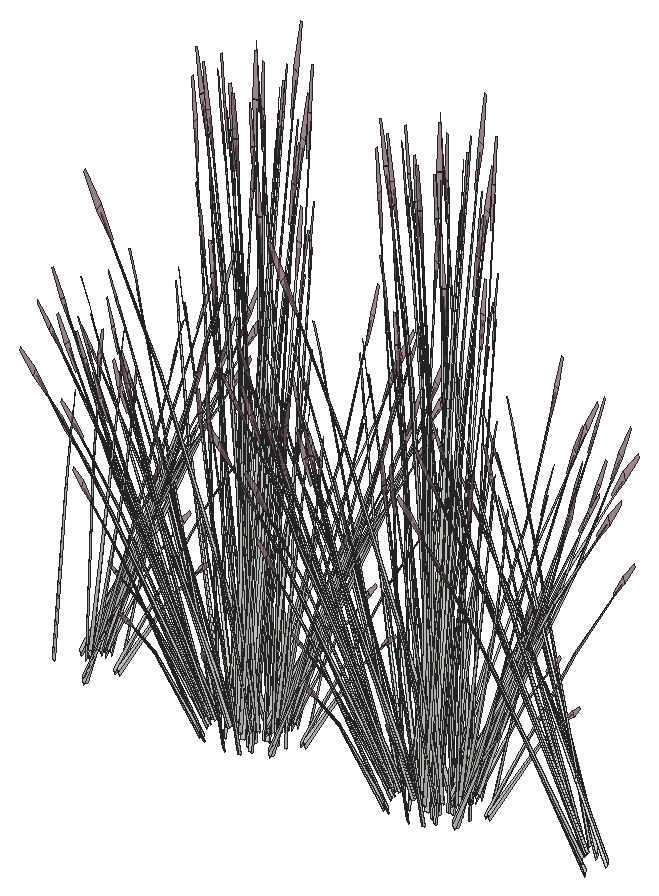
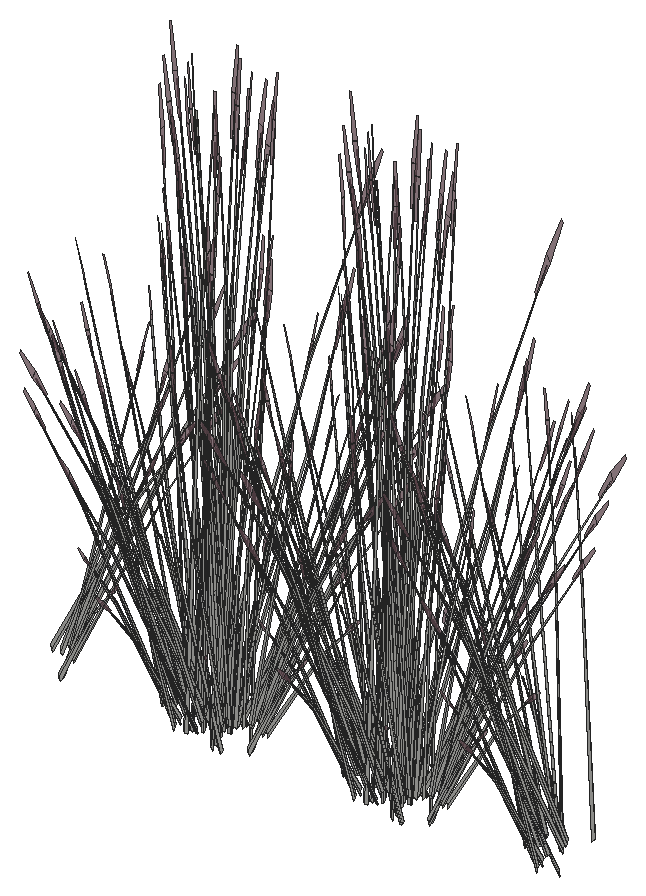
# SketchUp Ruby script. Lengths in inches.
U = 1.inch
M = Sketchup.active_model
def pt(a) = Geom::Point3d.new(a.map { |v| v * U })
def face(e, loops, mat)
  f = e.add_face(loops[0].map { |a| pt(a) })
  loops[1..].each { |l| e.add_face(l.map { |a| pt(a) }).erase! }
  f.material = f.back_material = mat if mat
  f
end
# faces: each face lists its corners as indices into pts; further lists are holes
def faces(e, pts, list, mat = nil) = list.each { |f| face(e, (f[0].is_a?(Array) ? f : [f]).map { |l| l.map { |i| pts[i] } }, mat) }
# xy, xz, yz: faces in a plane at the given z, y or x. An outline is a flat list of corners, or four numbers for a rectangle; further outlines are holes
def ring(l) = l.size == 4 ? [[l[0], l[1]], [l[2], l[1]], [l[2], l[3]], [l[0], l[3]]] : l.each_slice(2).to_a
def flat(e, list, mat, &to3) = list.each { |f| face(e, (f[0].is_a?(Array) ? f : [f]).map { |l| ring(l).map { |u, v| to3.(u, v) } }, mat) }
def xy(e, z, list, mat = nil) = flat(e, list, mat) { |x, y| [x, y, z] }
def xz(e, y, list, mat = nil) = flat(e, list, mat) { |x, z| [x, y, z] }
def yz(e, x, list, mat = nil) = flat(e, list, mat) { |y, z| [x, y, z] }
def lines(e, pts, list) = list.each { |a, b| e.add_line(pt(pts[a]), pt(pts[b])) }
# prism: a flat outline (further loops are holes) pulled along v
def prism(e, loops, v, mat = nil)
  f = face(e, loops, mat); d = Geom::Vector3d.new(v.map { |x| x * U })
  f.pushpull(f.normal.samedirection?(d) ? d.length : -d.length)
end
def box(e, o, s, mat = nil) = prism(e, [[o, [o[0] + s[0], o[1], o[2]], [o[0] + s[0], o[1] + s[1], o[2]], [o[0], o[1] + s[1], o[2]]]], [0, 0, s[2]], mat)
def at(x, y, z, deg = 0) = Geom::Transformation.translation(pt([x, y, z])) * Geom::Transformation.rotation(ORIGIN, Z_AXIS, deg.degrees)
def axes(o, x, y, z) = Geom::Transformation.new([*x, 0, *y, 0, *z, 0, *pt(o).to_a, 1])
def part(name) = M.definitions.add(name)
# library, detail: a bought-in or finely detailed component or shape, given as its bounding box
def library(name, o, s) = part(name).tap { |d| box(d.entities, o, s) }
def detail(e, o, s) = box(e.add_group.entities, o, s)
def put(e, d, t, mat = nil) = e.add_instance(d, t).tap { |i| i.material = mat if mat }
def group(e, t, mat = nil) = e.add_group.tap { |g| g.transformation = t; g.material = mat if mat }.entities
root = M.entities
M.materials.add("LightPink_Translucent").color = [144, 107, 117]
M.materials["LightPink_Translucent"].alpha = 0.75
c1 = part("blade")
p = [[2.15,0.21,22],[0,0.17,0],[0.09,0.45,0],[2.18,0.31,22],[2.29,0.31,22],[0.38,0.45,0],
  [2.48,0.24,33],[2.49,0.24,33],[2.48,0.22,33]]
faces(c1.entities,p,[[0,1,2,3],[4,5,2,3],[6,3,4,7],[8,0,3,6]])
c2 = part("seeds")
p = [[0.3,-0.1,1.38],[-0.01,-0.03,1.59],[-0.01,-0.03,0.03],[0.14,-0.07,-0.07],[0.29,-0.03,3],[0.15,0.01,3.11]]
faces(c2.entities,p,[[0,1,2,3],[1,0,4,5]],"LightPink_Translucent")
c3 = part("blade with seeds")
put(c3.entities,c1,at(0,0,0))
put(c3.entities,c2,axes([2.4,0.25,30.99],[1.5799,-0.05474,1.17369],[-0.12525,1.92788,0.29478],[-0.07173,-0.02425,1.56792]))
put(root,c3,axes([312.2,55.57,257.77],[-0.4278,-0.1757,1.1486],[0.5524,-0.17852,0.84392],[0.14899,0.15122,0.25299]))
put(root,c3,axes([310.68,55.38,257.59],[0.01341,-0.20255,1.43002],[0.64074,-0.22625,-0.30754],[0.1978,0.24243,0.61141]))
put(root,c3,axes([312.27,56.37,257.67],[-0.48723,-0.01916,1.0506],[0.32177,-0.40701,0.58006],[0.19248,0.1446,0.8241]))
put(root,c3,axes([310.8,51.49,258.875],[-0.14147,0.21002,1.71376],[-0.59349,-0.43464,0.13857],[0.26773,-0.27089,0.73262]))
put(root,c3,axes([311.24,55.8125,259.68],[0.74975,-0.14525,-0.51099],[0.13115,0.55007,-0.3958],[0.20138,0.15763,0.97773]))
put(root,c3,axes([312.7,52.53,259.68],[-0.19519,-0.55794,-0.51099],[0.73919,-0.0976,-0.3958],[0.21183,-0.14986,0.97773]))
put(root,c3,axes([314,55.41,258.93],[-0.14542,-0.51365,-0.03492],[0.68734,-0.11809,-0.15832],[0.14353,0.03256,0.52218]))
put(root,c3,axes([324.4375,52.72,258.875],[0.31515,-0.01384,1.71376],[-0.20907,0.5998,0.13857],[-0.44912,-0.0371,0.73262]))
put(root,c3,axes([313.6,51.42,257.77],[-0.25308,0.31105,1.1486],[-0.21753,-0.4179,0.84392],[0.20902,-0.10472,0.25299]))
put(root,c3,axes([311.16,54.37,258.875],[-0.28223,-0.10528,1.71376],[0.58406,-0.44165,0.13857],[0.36402,0.19924,0.73262]))
put(root,c3,axes([324.57,53.77,258.875],[0.26363,-0.12925,1.71376],[0.22195,0.59723,0.13857],[-0.41388,0.13498,0.73262]))
put(root,c3,axes([313.24,52.59,259.53],[0.66138,-0.08733,-0.35414],[0.17464,0.49921,0.4572],[0.18953,-0.13408,0.87481]))
put(root,c3,axes([323.75,54.79,257.59],[0.26405,0.05016,1.43002],[0.17019,0.51235,-0.30754],[-0.35868,0.0959,0.61141]))
put(root,c3,axes([312.72,52.76,259.98],[0.39688,-0.48213,-0.71045],[0.69548,0.34264,0.08574],[0.23697,-0.17468,1.00501]))
put(root,c3,axes([312.71,55.35,259.53],[0.43232,0.38257,-0.35414],[-0.49364,0.36215,0.4572],[0.25081,0.0551,0.87481]))
put(root,c3,axes([326.08,53.15,258.34],[0.21597,-0.08839,1.77064],[0.07448,0.61717,0.13857],[-0.4678,0.08189,0.63284]))
put(root,c3,axes([325.38,52.16,259.98],[-0.75952,-0.01471,-0.71045],[0.05101,-0.61953,0.08574],[-0.32177,-0.06538,1.00501]))
put(root,c3,axes([324.77,52.31,257.59],[0.14835,0.17012,1.43002],[-0.34183,0.46242,-0.30754],[-0.351,-0.11053,0.61141]))
put(root,c3,axes([313.04,53.77,259.68],[0.20584,-0.55581,-0.51099],[0.70573,0.19051,-0.3958],[0.28414,-0.05097,0.97773]))
put(root,c3,axes([324.16,53.23,259.53],[-0.63144,-0.17046,-0.35414],[0.18417,-0.49731,0.4572],[-0.25423,0.0456,0.87481]))
put(root,c3,axes([314.8125,54.125,257.77],[-0.46945,0.10088,1.1486],[0.22097,-0.4169,0.84392],[0.24904,0.02853,0.25299]))
put(root,c3,axes([325.03,51.75,258.875],[0.28223,0.10528,1.71376],[-0.58406,0.44165,0.13857],[-0.36402,-0.19924,0.73262]))
put(root,c3,axes([313.29,52.3125,257.59],[-0.27143,-0.0181,1.43002],[-0.27808,-0.48551,-0.30754],[0.33346,-0.13735,0.61141]))
put(root,c3,axes([313.47,54.02,259.53],[0.63144,0.17046,-0.35414],[-0.18417,0.49731,0.4572],[0.25423,-0.0456,0.87481]))
put(root,c3,axes([324.59,53.49,259.68],[-0.20584,0.55581,-0.51099],[-0.70573,-0.19051,-0.3958],[-0.28414,0.05097,0.97773]))
put(root,c3,axes([325.125,52.28,259.68],[-0.55171,0.40476,-0.51099],[-0.48318,-0.42758,-0.3958],[-0.28031,-0.06159,0.97773]))
put(root,c3,axes([312.25,55.1,259.98],[0.75952,0.01471,-0.71045],[-0.05101,0.61953,0.08574],[0.32177,0.06538,1.00501]))
put(root,c3,axes([311.75,53.41,258.875],[-0.31515,0.01384,1.71376],[0.20907,-0.5998,0.13857],[0.44912,0.0371,0.73262]))
put(root,c3,axes([323.2,55.86,257.77],[0.31665,-0.27694,1.1486],[0.12495,0.43841,0.84392],[-0.22883,0.0785,0.25299]))
put(root,c3,axes([312.91,53.97,259.98],[0.66765,-0.26986,-0.71045],[0.37208,0.55551,0.08574],[0.32259,-0.0631,1.00501]))
put(root,c3,axes([324.92,51.9,259.53],[-0.43232,-0.38257,-0.35414],[0.49364,-0.36215,0.4572],[-0.25081,-0.0551,0.87481]))
put(root,c3,axes([325.53,54.17,258.875],[0.18977,-0.18775,1.71376],[0.47917,0.50677,0.13857],[-0.32866,0.23079,0.73262]))
put(root,c3,axes([324.39,54.67,259.53],[-0.66138,0.08733,-0.35414],[-0.17464,-0.49921,0.4572],[-0.18953,0.13408,0.87481]))
put(root,c3,axes([323.88,52.82,257.77],[0.48508,-0.04372,1.1486],[-0.3077,0.38525,0.84392],[-0.23971,-0.05779,0.25299]))
put(root,c3,axes([313.93,54.79,257.59],[-0.18299,-0.15028,1.43002],[0.23809,-0.49714,-0.30754],[0.37023,0.06735,0.61141]))
put(root,c3,axes([325.39,54.64,258.875],[0.14147,-0.21002,1.71376],[0.59349,0.43464,0.13857],[-0.26773,0.27089,0.73262]))
put(root,c3,axes([324.94,54.72,259.68],[0.19519,0.55794,-0.51099],[-0.73919,0.0976,-0.3958],[-0.21183,0.14986,0.97773]))
put(root,c3,axes([326.7,51.43,259.98],[-0.64788,-0.29534,-0.71045],[0.46044,-0.51755,0.08574],[-0.23473,-0.17635,1.00501]))
put(root,c3,axes([326.4,51.44,259.68],[-0.74975,0.14525,-0.51099],[-0.13115,-0.55007,-0.3958],[-0.20138,-0.15763,0.97773]))
put(root,c3,axes([325.97,50.625,257.59],[-0.04601,0.19989,1.43002],[-0.67263,0.16733,-0.30754],[-0.15723,-0.25836,0.61141]))
put(root,c3,axes([326.19,51.14,258.875],[0.17368,0.19618,1.71376],[-0.80256,0.16516,0.13857],[-0.18139,-0.30799,0.73262]))
put(root,c3,axes([326.48,51.04,259.53],[-0.11735,-0.49217,-0.35414],[0.67083,-0.12996,0.4572],[-0.18018,-0.14104,0.87481]))
put(root,c3,axes([325.55,55.82,259.53],[-0.5141,0.32171,-0.35414],[-0.48666,-0.36734,0.4572],[-0.07405,0.18664,0.87481]))
put(root,c3,axes([328.25,54.77,258.33],[0.65659,0.2464,1.51261],[-0.64324,0.53082,0.59816],[-0.28812,-0.31461,1.26806]))
put(root,c3,axes([325.74,50.3,257.77],[0.39634,0.21267,1.1486],[-0.57721,0.12784,0.84392],[-0.1235,-0.16344,0.25299]))
put(root,c3,axes([325.88,57.07,257.77],[-0.01966,-0.36332,1.1486],[0.49135,0.25914,0.84392],[-0.09663,0.17317,0.25299]))
put(root,c3,axes([326.58,55.54,257.48],[0.7111,0.30552,0.49651],[-0.42504,0.54784,0],[-0.16196,-0.06958,1.57504]))
put(root,c3,axes([327.6,54.59,257.62],[-0.14658,0.54532,0.1448],[-0.71613,-0.09466,-0.41347],[-0.13033,-0.05599,1.26744]))
put(root,c3,axes([325.18,53.63,257.48],[0,0.61104,0.49651],[-0.85008,0,0],[0,-0.13917,1.57504]))
put(root,c3,axes([326.07,55.67,260],[0.54391,0.41056,-0.5672],[-0.57458,0.35956,-0.43934],[-0.08276,0.2086,1.08528]))
put(root,c3,axes([329.27,53.59,257.84],[-0.02076,-0.57531,1.41272],[0.93937,0.14913,0.59816],[-0.22217,0.31481,1.3335]))
put(root,c3,axes([325.47,56.29,257.82],[0.69024,-0.1082,0.06507],[0.15868,0.43593,-0.86304],[-0.04376,0.22067,0.7736]))
put(root,c3,axes([328.0625,51.1875,259.68],[-0.7469,-0.15318,-0.51099],[0.25601,-0.52518,-0.3958],[-0.06849,-0.21144,0.97773]))
put(root,c3,axes([327.37,54.07,257.36],[0.96033,0.12874,0.45755],[-0.19544,0.7271,0.17955],[-0.14034,-0.07021,1.58856]))
put(root,c3,axes([327.12,53.94,257.72],[-0.36864,0.55059,0.44739],[-0.76598,-0.26498,-0.21531],[0,-0.12692,1.43643]))
put(root,c3,axes([328.33,51.29,259.98],[-0.36264,-0.49684,-0.71045],[0.74649,-0.27689,0.08574],[-0.0848,-0.24006,1.00501]))
put(root,c3,axes([326.85,55.23,257.47],[0.81646,-0.16218,0.17642],[0.20161,0.60355,0.35086],[-0.07282,-0.08794,1.60407]))
put(root,c3,axes([329.28,55.27,257.47],[0.21949,-0.60727,0.17642],[0.8032,0.17185,0.35086],[-0.13875,0.00296,1.60407]))
put(root,c3,axes([328.91,54.46,257.62],[0.56134,0.36712,0.1448],[-0.46823,0.41419,-0.41347],[-0.13033,0.05599,1.26744]))
put(root,c3,axes([328.89,54.19,257.72],[0.82508,-0.03772,0.44739],[0.07462,0.62614,-0.21531],[-0.14771,0.06346,1.43643]))
put(root,c3,axes([329.51,55.59,257.48],[0.7111,-0.30552,0.49651],[0.42504,0.54784,0],[-0.16196,0.06958,1.57504]))
put(root,c3,axes([328.4,50.87,259.53],[0.22906,-0.4699,-0.35414],[0.66828,0.13705,0.4572],[-0.06128,-0.18919,0.87481]))
put(root,c3,axes([327.28,53.4,257.36],[0.33034,0.68327,0.45755],[-0.94388,0.2376,0.17955],[0.01154,-0.12555,1.58856]))
put(root,c3,axes([330.53,53.72,257.47],[-0.59697,-0.44509,0.17642],[0.60159,-0.4317,0.35086],[-0.06593,0.0909,1.60407]))
put(root,c3,axes([327.59,53.59,257.43],[0.8561,0.29616,0.24065],[-0.41201,0.61537,0.50002],[0,-0.14185,1.60543]))
put(root,c3,axes([327.3125,53.18,257.72],[-0.82508,0.03772,0.44739],[-0.07462,-0.62614,-0.21531],[0.14771,-0.06346,1.43643]))
put(root,c3,axes([326.93,52.1,257.47],[-0.21949,0.60727,0.17642],[-0.8032,-0.17185,0.35086],[0.13875,-0.00296,1.60407]))
put(root,c3,axes([329.36,52.14,257.47],[-0.81646,0.16218,0.17642],[-0.20161,-0.60355,0.35086],[0.07282,0.08794,1.60407]))
put(root,c3,axes([328.52,49.875,257.77],[0.09747,0.35631,1.1486],[-0.54071,-0.19735,0.84392],[0.05818,-0.18244,0.25299]))
put(root,c3,axes([328.02,53.02,257.36],[-0.62999,0.55453,0.45755],[-0.74845,-0.4895,0.17955],[0.15188,-0.05534,1.58856]))
put(root,c3,axes([329.09,53.43,257.72],[0.36864,-0.55059,0.44739],[0.76598,0.26498,-0.21531],[0,0.12692,1.43643]))
put(root,c3,axes([327.68,56.07,259.68],[0.7469,0.15318,-0.51099],[-0.25601,0.52518,-0.3958],[0.06849,0.21144,0.97773]))
put(root,c3,axes([328.84,53.3,257.38],[-0.96033,-0.12874,0.49198],[0.19544,-0.7271,0.19306],[0.14034,0.07021,1.70813]))
put(root,c3,axes([328.3,52.92,257.72],[-0.45644,-0.51287,0.44739],[0.69137,-0.36116,-0.21531],[0.14771,0.06346,1.43643]))
put(root,c3,axes([329.41,53.55,257.62],[0.70791,-0.1782,0.1448],[0.24791,0.50885,-0.41347],[0,0.11199,1.26744]))
put(root,c3,axes([329.67,51.59,259.68],[-0.54391,-0.41056,-0.51099],[0.57458,-0.35956,-0.3958],[0.08276,-0.2086,0.97773]))
put(root,c3,axes([329.32,50.86,257.59],[-0.21597,0.12368,1.43002],[-0.64681,-0.21647,-0.30754],[0.1199,-0.26922,0.61141]))
put(root,c3,axes([331.02,53.74,257.48],[0,-0.61104,0.49651],[0.85008,0,0],[0,0.13917,1.57504]))
put(root,c3,axes([328.1,54.98,258.875],[-0.17368,-0.19618,1.71376],[0.80256,-0.16516,0.13857],[0.18139,0.30799,0.73262]))
put(root,c3,axes([328.6,52.78,257.62],[0.14658,-0.54532,0.1448],[0.71613,0.09466,-0.41347],[0.13033,0.05599,1.26744]))
put(root,c3,axes([329.62,51.83,257.48],[-0.7111,-0.30552,0.49651],[0.42504,-0.54784,0],[0.16196,0.06958,1.57504]))
put(root,c3,axes([329.84,51.77,259.98],[0.01977,-0.56521,-0.71045],[0.83252,0.03796,0.08574],[0.08786,-0.23945,1.00501]))
put(root,c3,axes([330.1875,51.43,259.53],[0.5141,-0.32171,-0.35414],[0.48666,0.36734,0.4572],[0.07405,-0.18664,0.87481]))
put(root,c3,axes([330.31,55.57,257.77],[-0.4278,-0.1757,1.1486],[0.5524,-0.17852,0.84392],[0.14899,0.15122,0.25299]))
put(root,c3,axes([328.79,55.38,257.59],[0.01341,-0.20255,1.43002],[0.64074,-0.22625,-0.30754],[0.1978,0.24243,0.61141]))
put(root,c3,axes([330.38,56.37,257.67],[-0.48723,-0.01916,1.0506],[0.32177,-0.40701,0.58006],[0.19248,0.1446,0.8241]))
put(root,c3,axes([328.91,51.49,258.875],[-0.14147,0.21002,1.71376],[-0.59349,-0.43464,0.13857],[0.26773,-0.27089,0.73262]))
put(root,c3,axes([329.34,55.8125,259.68],[0.74975,-0.14525,-0.51099],[0.13115,0.55007,-0.3958],[0.20138,0.15763,0.97773]))
put(root,c3,axes([330.8,52.53,259.68],[-0.19519,-0.55794,-0.51099],[0.73919,-0.0976,-0.3958],[0.21183,-0.14986,0.97773]))
put(root,c3,axes([342.34,52.72,258.875],[0.31515,-0.01384,1.71376],[-0.20907,0.5998,0.13857],[-0.44912,-0.0371,0.73262]))
put(root,c3,axes([332.1,55.41,258.93],[-0.14542,-0.51365,-0.03492],[0.68734,-0.11809,-0.15832],[0.14353,0.03256,0.52218]))
put(root,c3,axes([331.71,51.42,257.77],[-0.25308,0.31105,1.1486],[-0.21753,-0.4179,0.84392],[0.20902,-0.10472,0.25299]))
put(root,c3,axes([342.47,53.77,258.875],[0.26363,-0.12925,1.71376],[0.22195,0.59723,0.13857],[-0.41388,0.13498,0.73262]))
put(root,c3,axes([329.26,54.37,258.875],[-0.28223,-0.10528,1.71376],[0.58406,-0.44165,0.13857],[0.36402,0.19924,0.73262]))
put(root,c3,axes([341.65,54.79,257.59],[0.26405,0.05016,1.43002],[0.17019,0.51235,-0.30754],[-0.35868,0.0959,0.61141]))
put(root,c3,axes([331.35,52.59,259.53],[0.66138,-0.08733,-0.35414],[0.17464,0.49921,0.4572],[0.18953,-0.13408,0.87481]))
put(root,c3,axes([330.82,52.76,259.98],[0.39688,-0.48213,-0.71045],[0.69548,0.34264,0.08574],[0.23697,-0.17468,1.00501]))
put(root,c3,axes([343.99,53.15,258.34],[0.21597,-0.08839,1.77064],[0.07448,0.61717,0.13857],[-0.4678,0.08189,0.63284]))
put(root,c3,axes([330.82,55.35,259.53],[0.43232,0.38257,-0.35414],[-0.49364,0.36215,0.4572],[0.25081,0.0551,0.87481]))
put(root,c3,axes([343.29,52.16,259.98],[-0.75952,-0.01471,-0.71045],[0.05101,-0.61953,0.08574],[-0.32177,-0.06538,1.00501]))
put(root,c3,axes([342.67,52.31,257.59],[0.14835,0.17012,1.43002],[-0.34183,0.46242,-0.30754],[-0.351,-0.11053,0.61141]))
put(root,c3,axes([342.06,53.23,259.53],[-0.63144,-0.17046,-0.35414],[0.18417,-0.49731,0.4572],[-0.25423,0.0456,0.87481]))
put(root,c3,axes([342.9375,51.75,258.875],[0.28223,0.10528,1.71376],[-0.58406,0.44165,0.13857],[-0.36402,-0.19924,0.73262]))
put(root,c3,axes([331.15,53.77,259.68],[0.20584,-0.55581,-0.51099],[0.70573,0.19051,-0.3958],[0.28414,-0.05097,0.97773]))
put(root,c3,axes([332.92,54.125,257.77],[-0.46945,0.10088,1.1486],[0.22097,-0.4169,0.84392],[0.24904,0.02853,0.25299]))
put(root,c3,axes([342.5,53.49,259.68],[-0.20584,0.55581,-0.51099],[-0.70573,-0.19051,-0.3958],[-0.28414,0.05097,0.97773]))
put(root,c3,axes([331.4,52.3125,257.59],[-0.27143,-0.0181,1.43002],[-0.27808,-0.48551,-0.30754],[0.33346,-0.13735,0.61141]))
put(root,c3,axes([331.58,54.02,259.53],[0.63144,0.17046,-0.35414],[-0.18417,0.49731,0.4572],[0.25423,-0.0456,0.87481]))
put(root,c3,axes([343.03,52.28,259.68],[-0.55171,0.40476,-0.51099],[-0.48318,-0.42758,-0.3958],[-0.28031,-0.06159,0.97773]))
put(root,c3,axes([330.36,55.1,259.98],[0.75952,0.01471,-0.71045],[-0.05101,0.61953,0.08574],[0.32177,0.06538,1.00501]))
put(root,c3,axes([341.1,55.86,257.77],[0.31665,-0.27694,1.1486],[0.12495,0.43841,0.84392],[-0.22883,0.0785,0.25299]))
put(root,c3,axes([329.86,53.41,258.875],[-0.31515,0.01384,1.71376],[0.20907,-0.5998,0.13857],[0.44912,0.0371,0.73262]))
put(root,c3,axes([342.83,51.9,259.53],[-0.43232,-0.38257,-0.35414],[0.49364,-0.36215,0.4572],[-0.25081,-0.0551,0.87481]))
put(root,c3,axes([343.4375,54.17,258.875],[0.18977,-0.18775,1.71376],[0.47917,0.50677,0.13857],[-0.32866,0.23079,0.73262]))
put(root,c3,axes([342.3,54.67,259.53],[-0.66138,0.08733,-0.35414],[-0.17464,-0.49921,0.4572],[-0.18953,0.13408,0.87481]))
put(root,c3,axes([331.01,53.97,259.98],[0.66765,-0.26986,-0.71045],[0.37208,0.55551,0.08574],[0.32259,-0.0631,1.00501]))
put(root,c3,axes([341.79,52.82,257.77],[0.48508,-0.04372,1.1486],[-0.3077,0.38525,0.84392],[-0.23971,-0.05779,0.25299]))
put(root,c3,axes([332.04,54.79,257.59],[-0.18299,-0.15028,1.43002],[0.23809,-0.49714,-0.30754],[0.37023,0.06735,0.61141]))
put(root,c3,axes([343.3,54.64,258.875],[0.14147,-0.21002,1.71376],[0.59349,0.43464,0.13857],[-0.26773,0.27089,0.73262]))
put(root,c3,axes([342.84,54.72,259.68],[0.19519,0.55794,-0.51099],[-0.73919,0.0976,-0.3958],[-0.21183,0.14986,0.97773]))
put(root,c3,axes([344.61,51.43,259.98],[-0.64788,-0.29534,-0.71045],[0.46044,-0.51755,0.08574],[-0.23473,-0.17635,1.00501]))
put(root,c3,axes([344.3,51.44,259.68],[-0.74975,0.14525,-0.51099],[-0.13115,-0.55007,-0.3958],[-0.20138,-0.15763,0.97773]))
put(root,c3,axes([343.88,50.625,257.59],[-0.04601,0.19989,1.43002],[-0.67263,0.16733,-0.30754],[-0.15723,-0.25836,0.61141]))
put(root,c3,axes([344.1,51.14,258.875],[0.17368,0.19618,1.71376],[-0.80256,0.16516,0.13857],[-0.18139,-0.30799,0.73262]))
put(root,c3,axes([344.38,51.04,259.53],[-0.11735,-0.49217,-0.35414],[0.67083,-0.12996,0.4572],[-0.18018,-0.14104,0.87481]))
put(root,c3,axes([343.46,55.82,259.53],[-0.5141,0.32171,-0.35414],[-0.48666,-0.36734,0.4572],[-0.07405,0.18664,0.87481]))
put(root,c3,axes([346.16,54.77,258.33],[0.65659,0.2464,1.51261],[-0.64324,0.53082,0.59816],[-0.28812,-0.31461,1.26806]))
put(root,c3,axes([343.65,50.3,257.77],[0.39634,0.21267,1.1486],[-0.57721,0.12784,0.84392],[-0.1235,-0.16344,0.25299]))
put(root,c3,axes([343.79,57.07,257.77],[-0.01966,-0.36332,1.1486],[0.49135,0.25914,0.84392],[-0.09663,0.17317,0.25299]))
put(root,c3,axes([344.49,55.54,257.48],[0.7111,0.30552,0.49651],[-0.42504,0.54784,0],[-0.16196,-0.06958,1.57504]))
put(root,c3,axes([345.51,54.59,257.62],[-0.14658,0.54532,0.1448],[-0.71613,-0.09466,-0.41347],[-0.13033,-0.05599,1.26744]))
put(root,c3,axes([343.09,53.63,257.48],[0,0.61104,0.49651],[-0.85008,0,0],[0,-0.13917,1.57504]))
put(root,c3,axes([343.97,55.67,260],[0.54391,0.41056,-0.5672],[-0.57458,0.35956,-0.43934],[-0.08276,0.2086,1.08528]))
put(root,c3,axes([347.17,53.59,257.84],[-0.02076,-0.57531,1.41272],[0.93937,0.14913,0.59816],[-0.22217,0.31481,1.3335]))
put(root,c3,axes([343.38,56.29,257.82],[0.69024,-0.1082,0.06507],[0.15868,0.43593,-0.86304],[-0.04376,0.22067,0.7736]))
put(root,c3,axes([345.97,51.1875,259.68],[-0.7469,-0.15318,-0.51099],[0.25601,-0.52518,-0.3958],[-0.06849,-0.21144,0.97773]))
put(root,c3,axes([345.27,54.07,257.36],[0.96033,0.12874,0.45755],[-0.19544,0.7271,0.17955],[-0.14034,-0.07021,1.58856]))
put(root,c3,axes([345.02,53.94,257.72],[-0.36864,0.55059,0.44739],[-0.76598,-0.26498,-0.21531],[0,-0.12692,1.43643]))
put(root,c3,axes([346.24,51.29,259.98],[-0.36264,-0.49684,-0.71045],[0.74649,-0.27689,0.08574],[-0.0848,-0.24006,1.00501]))
put(root,c3,axes([344.76,55.23,257.47],[0.81646,-0.16218,0.17642],[0.20161,0.60355,0.35086],[-0.07282,-0.08794,1.60407]))
put(root,c3,axes([347.1875,55.27,257.47],[0.21949,-0.60727,0.17642],[0.8032,0.17185,0.35086],[-0.13875,0.00296,1.60407]))
put(root,c3,axes([346.81,54.46,257.62],[0.56134,0.36712,0.1448],[-0.46823,0.41419,-0.41347],[-0.13033,0.05599,1.26744]))
put(root,c3,axes([346.8,54.19,257.72],[0.82508,-0.03772,0.44739],[0.07462,0.62614,-0.21531],[-0.14771,0.06346,1.43643]))
put(root,c3,axes([347.41,55.59,257.48],[0.7111,-0.30552,0.49651],[0.42504,0.54784,0],[-0.16196,0.06958,1.57504]))
put(root,c3,axes([346.31,50.87,259.53],[0.22906,-0.4699,-0.35414],[0.66828,0.13705,0.4572],[-0.06128,-0.18919,0.87481]))
put(root,c3,axes([345.1875,53.4,257.36],[0.33034,0.68327,0.45755],[-0.94388,0.2376,0.17955],[0.01154,-0.12555,1.58856]))
put(root,c3,axes([348.4375,53.72,257.47],[-0.59697,-0.44509,0.17642],[0.60159,-0.4317,0.35086],[-0.06593,0.0909,1.60407]))
put(root,c3,axes([345.49,53.59,257.43],[0.8561,0.29616,0.24065],[-0.41201,0.61537,0.50002],[0,-0.14185,1.60543]))
put(root,c3,axes([345.22,53.18,257.72],[-0.82508,0.03772,0.44739],[-0.07462,-0.62614,-0.21531],[0.14771,-0.06346,1.43643]))
put(root,c3,axes([344.83,52.1,257.47],[-0.21949,0.60727,0.17642],[-0.8032,-0.17185,0.35086],[0.13875,-0.00296,1.60407]))
put(root,c3,axes([347.26,52.14,257.47],[-0.81646,0.16218,0.17642],[-0.20161,-0.60355,0.35086],[0.07282,0.08794,1.60407]))
put(root,c3,axes([346.43,49.875,257.77],[0.09747,0.35631,1.1486],[-0.54071,-0.19735,0.84392],[0.05818,-0.18244,0.25299]))
put(root,c3,axes([345.93,53.02,257.36],[-0.62999,0.55453,0.45755],[-0.74845,-0.4895,0.17955],[0.15188,-0.05534,1.58856]))
put(root,c3,axes([347,53.43,257.72],[0.36864,-0.55059,0.44739],[0.76598,0.26498,-0.21531],[0,0.12692,1.43643]))
put(root,c3,axes([345.58,56.07,259.68],[0.7469,0.15318,-0.51099],[-0.25601,0.52518,-0.3958],[0.06849,0.21144,0.97773]))
put(root,c3,axes([346.75,53.3,257.38],[-0.96033,-0.12874,0.49198],[0.19544,-0.7271,0.19306],[0.14034,0.07021,1.70813]))
put(root,c3,axes([346.2,52.92,257.72],[-0.45644,-0.51287,0.44739],[0.69137,-0.36116,-0.21531],[0.14771,0.06346,1.43643]))
put(root,c3,axes([347.32,53.55,257.62],[0.70791,-0.1782,0.1448],[0.24791,0.50885,-0.41347],[0,0.11199,1.26744]))
put(root,c3,axes([347.58,51.59,259.68],[-0.54391,-0.41056,-0.51099],[0.57458,-0.35956,-0.3958],[0.08276,-0.2086,0.97773]))
put(root,c3,axes([347.22,50.86,257.59],[-0.21597,0.12368,1.43002],[-0.64681,-0.21647,-0.30754],[0.1199,-0.26922,0.61141]))
put(root,c3,axes([348.93,53.74,257.48],[0,-0.61104,0.49651],[0.85008,0,0],[0,0.13917,1.57504]))
put(root,c3,axes([346.01,54.98,258.875],[-0.17368,-0.19618,1.71376],[0.80256,-0.16516,0.13857],[0.18139,0.30799,0.73262]))
put(root,c3,axes([346.51,52.78,257.62],[0.14658,-0.54532,0.1448],[0.71613,0.09466,-0.41347],[0.13033,0.05599,1.26744]))
put(root,c3,axes([347.53,51.83,257.48],[-0.7111,-0.30552,0.49651],[0.42504,-0.54784,0],[0.16196,0.06958,1.57504]))
put(root,c3,axes([347.75,51.77,259.98],[0.01977,-0.56521,-0.71045],[0.83252,0.03796,0.08574],[0.08786,-0.23945,1.00501]))
put(root,c3,axes([348.09,51.43,259.53],[0.5141,-0.32171,-0.35414],[0.48666,0.36734,0.4572],[0.07405,-0.18664,0.87481]))
put(root,c3,axes([348.22,55.57,257.77],[-0.4278,-0.1757,1.1486],[0.5524,-0.17852,0.84392],[0.14899,0.15122,0.25299]))
put(root,c3,axes([346.69,55.38,257.59],[0.01341,-0.20255,1.43002],[0.64074,-0.22625,-0.30754],[0.1978,0.24243,0.61141]))
put(root,c3,axes([348.28,56.37,257.67],[-0.48723,-0.01916,1.0506],[0.32177,-0.40701,0.58006],[0.19248,0.1446,0.8241]))
put(root,c3,axes([346.8125,51.49,258.875],[-0.14147,0.21002,1.71376],[-0.59349,-0.43464,0.13857],[0.26773,-0.27089,0.73262]))
put(root,c3,axes([347.25,55.8125,259.68],[0.74975,-0.14525,-0.51099],[0.13115,0.55007,-0.3958],[0.20138,0.15763,0.97773]))
put(root,c3,axes([348.71,52.53,259.68],[-0.19519,-0.55794,-0.51099],[0.73919,-0.0976,-0.3958],[0.21183,-0.14986,0.97773]))
put(root,c3,axes([350.01,55.41,258.93],[-0.14542,-0.51365,-0.03492],[0.68734,-0.11809,-0.15832],[0.14353,0.03256,0.52218]))
put(root,c3,axes([349.62,51.42,257.77],[-0.25308,0.31105,1.1486],[-0.21753,-0.4179,0.84392],[0.20902,-0.10472,0.25299]))
put(root,c3,axes([361.125,52.72,258.875],[0.31515,-0.01384,1.71376],[-0.20907,0.5998,0.13857],[-0.44912,-0.0371,0.73262]))
put(root,c3,axes([347.17,54.37,258.875],[-0.28223,-0.10528,1.71376],[0.58406,-0.44165,0.13857],[0.36402,0.19924,0.73262]))
put(root,c3,axes([349.26,52.59,259.53],[0.66138,-0.08733,-0.35414],[0.17464,0.49921,0.4572],[0.18953,-0.13408,0.87481]))
put(root,c3,axes([348.73,52.76,259.98],[0.39688,-0.48213,-0.71045],[0.69548,0.34264,0.08574],[0.23697,-0.17468,1.00501]))
put(root,c3,axes([348.72,55.35,259.53],[0.43232,0.38257,-0.35414],[-0.49364,0.36215,0.4572],[0.25081,0.0551,0.87481]))
put(root,c3,axes([361.26,53.77,258.875],[0.26363,-0.12925,1.71376],[0.22195,0.59723,0.13857],[-0.41388,0.13498,0.73262]))
put(root,c3,axes([360.44,54.79,257.59],[0.26405,0.05016,1.43002],[0.17019,0.51235,-0.30754],[-0.35868,0.0959,0.61141]))
put(root,c3,axes([362.77,53.15,258.34],[0.21597,-0.08839,1.77064],[0.07448,0.61717,0.13857],[-0.4678,0.08189,0.63284]))
put(root,c3,axes([349.05,53.77,259.68],[0.20584,-0.55581,-0.51099],[0.70573,0.19051,-0.3958],[0.28414,-0.05097,0.97773]))
put(root,c3,axes([350.83,54.125,257.77],[-0.46945,0.10088,1.1486],[0.22097,-0.4169,0.84392],[0.24904,0.02853,0.25299]))
put(root,c3,axes([349.31,52.3125,257.59],[-0.27143,-0.0181,1.43002],[-0.27808,-0.48551,-0.30754],[0.33346,-0.13735,0.61141]))
put(root,c3,axes([349.49,54.02,259.53],[0.63144,0.17046,-0.35414],[-0.18417,0.49731,0.4572],[0.25423,-0.0456,0.87481]))
put(root,c3,axes([362.07,52.16,259.98],[-0.75952,-0.01471,-0.71045],[0.05101,-0.61953,0.08574],[-0.32177,-0.06538,1.00501]))
put(root,c3,axes([348.27,55.1,259.98],[0.75952,0.01471,-0.71045],[-0.05101,0.61953,0.08574],[0.32177,0.06538,1.00501]))
put(root,c3,axes([361.46,52.31,257.59],[0.14835,0.17012,1.43002],[-0.34183,0.46242,-0.30754],[-0.351,-0.11053,0.61141]))
put(root,c3,axes([360.85,53.23,259.53],[-0.63144,-0.17046,-0.35414],[0.18417,-0.49731,0.4572],[-0.25423,0.0456,0.87481]))
put(root,c3,axes([361.72,51.75,258.875],[0.28223,0.10528,1.71376],[-0.58406,0.44165,0.13857],[-0.36402,-0.19924,0.73262]))
put(root,c3,axes([347.77,53.41,258.875],[-0.31515,0.01384,1.71376],[0.20907,-0.5998,0.13857],[0.44912,0.0371,0.73262]))
put(root,c3,axes([361.28,53.49,259.68],[-0.20584,0.55581,-0.51099],[-0.70573,-0.19051,-0.3958],[-0.28414,0.05097,0.97773]))
put(root,c3,axes([348.92,53.97,259.98],[0.66765,-0.26986,-0.71045],[0.37208,0.55551,0.08574],[0.32259,-0.0631,1.00501]))
put(root,c3,axes([361.82,52.28,259.68],[-0.55171,0.40476,-0.51099],[-0.48318,-0.42758,-0.3958],[-0.28031,-0.06159,0.97773]))
put(root,c3,axes([359.88,55.86,257.77],[0.31665,-0.27694,1.1486],[0.12495,0.43841,0.84392],[-0.22883,0.0785,0.25299]))
put(root,c3,axes([349.95,54.79,257.59],[-0.18299,-0.15028,1.43002],[0.23809,-0.49714,-0.30754],[0.37023,0.06735,0.61141]))
